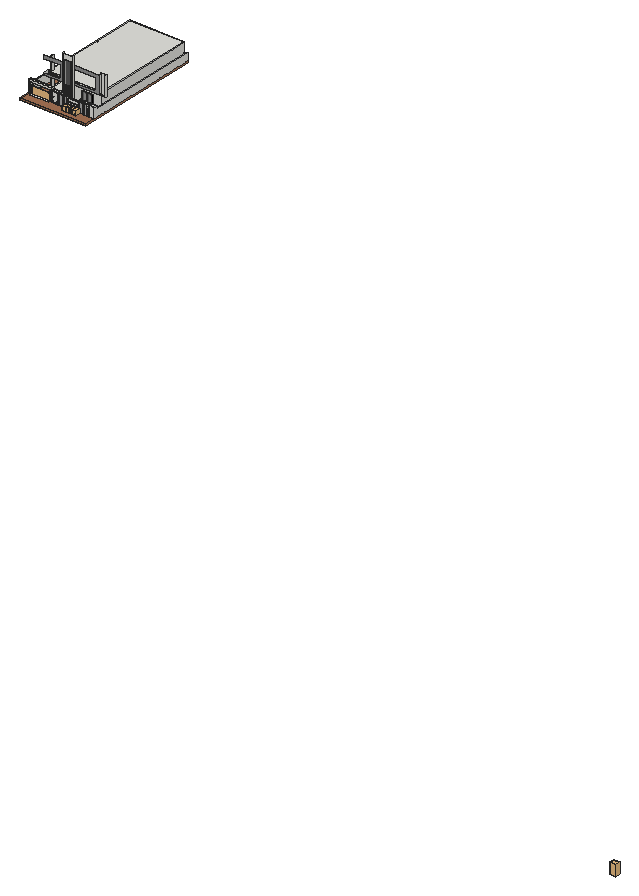
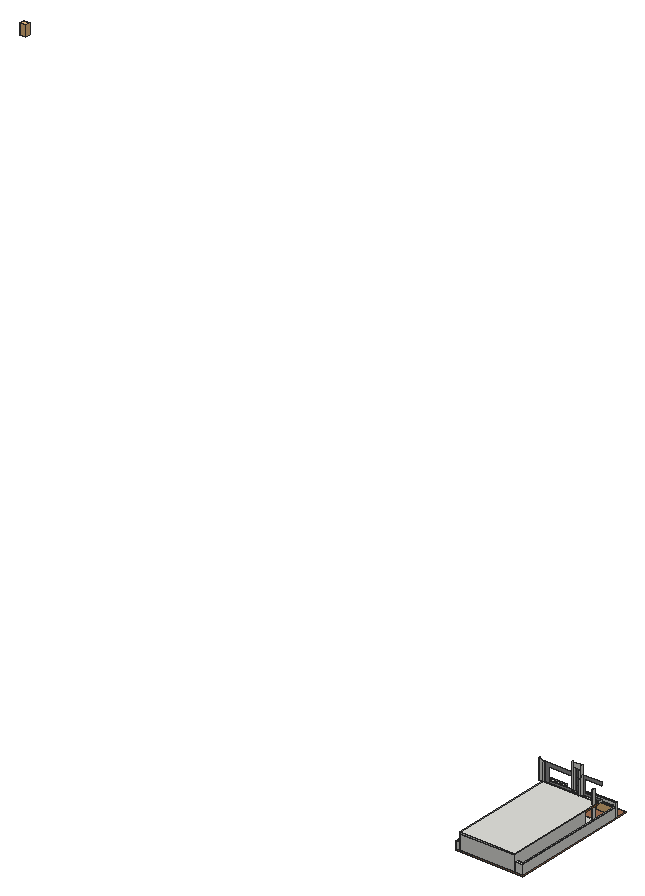
# SketchUp Ruby script. Lengths in inches.
U = 1.inch
M = Sketchup.active_model
def pt(a) = Geom::Point3d.new(a.map { |v| v * U })
def face(e, loops, mat)
  f = e.add_face(loops[0].map { |a| pt(a) })
  loops[1..].each { |l| e.add_face(l.map { |a| pt(a) }).erase! }
  f.material = f.back_material = mat if mat
  f
end
# faces: each face lists its corners as indices into pts; further lists are holes
def faces(e, pts, list, mat = nil) = list.each { |f| face(e, (f[0].is_a?(Array) ? f : [f]).map { |l| l.map { |i| pts[i] } }, mat) }
# xy, xz, yz: faces in a plane at the given z, y or x. An outline is a flat list of corners, or four numbers for a rectangle; further outlines are holes
def ring(l) = l.size == 4 ? [[l[0], l[1]], [l[2], l[1]], [l[2], l[3]], [l[0], l[3]]] : l.each_slice(2).to_a
def flat(e, list, mat, &to3) = list.each { |f| face(e, (f[0].is_a?(Array) ? f : [f]).map { |l| ring(l).map { |u, v| to3.(u, v) } }, mat) }
def xy(e, z, list, mat = nil) = flat(e, list, mat) { |x, y| [x, y, z] }
def xz(e, y, list, mat = nil) = flat(e, list, mat) { |x, z| [x, y, z] }
def yz(e, x, list, mat = nil) = flat(e, list, mat) { |y, z| [x, y, z] }
def lines(e, pts, list) = list.each { |a, b| e.add_line(pt(pts[a]), pt(pts[b])) }
# prism: a flat outline (further loops are holes) pulled along v
def prism(e, loops, v, mat = nil)
  f = face(e, loops, mat); d = Geom::Vector3d.new(v.map { |x| x * U })
  f.pushpull(f.normal.samedirection?(d) ? d.length : -d.length)
end
def box(e, o, s, mat = nil) = prism(e, [[o, [o[0] + s[0], o[1], o[2]], [o[0] + s[0], o[1] + s[1], o[2]], [o[0], o[1] + s[1], o[2]]]], [0, 0, s[2]], mat)
def at(x, y, z, deg = 0) = Geom::Transformation.translation(pt([x, y, z])) * Geom::Transformation.rotation(ORIGIN, Z_AXIS, deg.degrees)
def axes(o, x, y, z) = Geom::Transformation.new([*x, 0, *y, 0, *z, 0, *pt(o).to_a, 1])
def part(name) = M.definitions.add(name)
# library, detail: a bought-in or finely detailed component or shape, given as its bounding box
def library(name, o, s) = part(name).tap { |d| box(d.entities, o, s) }
def detail(e, o, s) = box(e.add_group.entities, o, s)
def put(e, d, t, mat = nil) = e.add_instance(d, t).tap { |i| i.material = mat if mat }
def group(e, t, mat = nil) = e.add_group.tap { |g| g.transformation = t; g.material = mat if mat }.entities
root = M.entities
M.materials.add("[Color B02]").color = [255, 178, 153]
M.materials.add("[Color M03]").color = [170, 170, 170]
M.materials.add("[Color M04]").color = [142, 142, 142]
M.materials.add("[Color M08]").color = [30, 30, 30]
M.materials.add("[Color_008]").color = [30, 30, 30]
M.materials.add("[Color_009]").color = [0, 0, 0]
M.materials.add("[Granite Dark Gray]").color = [69, 68, 68]
M.materials.add("[Tile Ceramic Multi]").color = [165, 115, 84]
M.materials.add("[Translucent Glass Gray]1").color = [128, 128, 128]
M.materials["[Translucent Glass Gray]1"].alpha = 0.5
M.materials.add("[Translucent_Glass_Gray]").color = [128, 128, 128]
M.materials["[Translucent_Glass_Gray]"].alpha = 0.5
M.materials.add("[Wood Bamboo]").color = [177, 105, 43]
c1 = library("climbing plant",[8874.76,-5589.78,-33.625],[50.13,38.07,87.16])
c2 = library("Slatted driveway gate",[-314.09,973.28,-346.04],[148.54,5.33,60.07])
c3 = part("Group\#12")
xz(c3.entities,0,[[0,0,51.1875,2.08]])
c4 = library("Broadleaf plant",[0,0,0],[149.19,166.1,98.1875])
c5 = part("Group\#13")
xz(c5.entities,0,[[0,0,45.4375,2.7]])
c6 = part("Janela")
xy(c6.entities,0,[[96.33,43.17,179.01,44.35]],"[Color_009]")
xy(c6.entities,1.97,[[98.3,44.15,136.6875,44.35],[138.66,44.15,177.04,44.35]])
xy(c6.entities,1.97,[[98.3,43.17,136.6875,43.46],[138.66,43.17,177.04,43.46]],"[Color_009]")
xy(c6.entities,80.71,[[98.3,43.17,136.6875,43.46],[138.66,43.17,177.04,43.46],[98.3,43.46,136.6875,44.15],[138.66,43.46,177.04,44.15],[98.3,44.15,136.6875,44.35],
  [138.66,44.15,177.04,44.35]])
xy(c6.entities,82.68,[[96.33,43.17,179.01,44.35]],"[Color_008]")
xz(c6.entities,43.17,[[[96.33,0,179.01,82.68],[98.3,1.97,136.6875,80.71],[138.66,1.97,177.04,80.71]]],"[Color_009]")
xz(c6.entities,43.46,[[98.3,1.97,136.6875,80.71],[138.66,1.97,177.04,80.71]],"[Translucent_Glass_Gray]")
xz(c6.entities,44.15,[[98.3,1.97,136.6875,80.71],[138.66,1.97,177.04,80.71]],"[Translucent_Glass_Gray]")
xz(c6.entities,44.35,[[[96.33,0,179.01,82.68],[98.3,1.97,177.04,80.71]],[136.6875,1.97,138.66,80.71]],"[Color_009]")
yz(c6.entities,96.33,[[43.17,0,44.35,82.68]],"[Color_009]")
yz(c6.entities,98.3,[[44.15,1.97,44.35,80.71]])
yz(c6.entities,98.3,[[43.17,1.97,43.46,80.71]],"[Color_009]")
yz(c6.entities,136.6875,[[43.17,1.97,43.46,80.71],[44.15,1.97,44.35,80.71]],"[Color_009]")
yz(c6.entities,138.66,[[43.17,1.97,43.46,80.71],[44.15,1.97,44.35,80.71]])
yz(c6.entities,177.04,[[43.17,1.97,43.46,80.71],[44.15,1.97,44.35,80.71]],"[Color_009]")
yz(c6.entities,179.01,[[43.17,0,44.35,82.68]],"[Color_009]")
c7 = library("Aluprof_MB-86_Drzwi_panelowe_003_S-0452",[0,0,0],[44.84,5.36,87])
c8 = part("Group\#15")
xz(c8.entities,0,[[0,0,96.8125,17.4]])
c9 = part("Group\#5")
box(c9.entities,[0,-1.25,0],[78.66,1.25,2.55])
c10 = part("Group\#6")
box(c10.entities,[0,-1.25,0],[15.54,1.25,1.96])
c11 = part("Group\#7")
box(c11.entities,[0,-1.25,0],[16.29,1.25,1.96])
c12 = part("Group\#10")
prism(c12.entities,[[[0,0.01,-2.4375],[0,129.01,-2.125],[7.8,129.01,-2.125],[7.8,0.01,-2.4375]]],[0,-0.01,2.4375])
xy(root,-0.4375,[[[316.25,46.4375,413.0625,87.8125],[320.83,51.02,408.48,83.23]],[320.83,51.02,408.48,83.23],[17.8125,71.9,174.3125,87.8125],[192.625,83.75,243.8125,107],[252.5625,83.75,280.625,107],
  [289.375,83.75,316.25,107],[413.0625,83.75,443.75,107],[452.5625,83.75,482.4375,107],[493.1875,83.75,493.1875,107,527.125,107,527.125,1033.27,506,1033.27,506,1045,538.625,1045,538.625,83.75],[0,87.8125,17.8125,104.375],
  [174.08,87.8125,192.625,104.375],[243.8125,87.8125,252.5625,107],[280.625,87.8125,289.375,107],[316.25,87.8125,413.0625,107],[443.75,87.8125,452.5625,107],
  [482.4375,87.8125,493.1875,107],[0,104.375,0,1045,62,1045,62,1019.26,13.64,1019.26,13.64,104.375],[[62,205,62,1045,505.75,1045,505.75,1033.27,506,1033.27,506,205],[71,214,497,214,497,518,353,518,353,338,349,338,349,522,397,522,397,582,349,582,349,758,418,758,418,806,373,806,373,936,237,936,237,864,183,864,183,734,179,734,179,800,71,800,71,526,239,526,239,730,243,730,243,522,219,522,219,338,71,338],[71,868,233,1036],[71,342,215,522],[353,586,497,754],[377,892,497,1036],[377,810,497,888],[301,940,373,1036],[71,804,179,864],[237,940,297,1036],[401,522,497,582],[422,758,497,806]],[505.75,1033.27,506,1045]])
xy(root,0,[[62,205,71,205,71,225.73,68.72,225.73,68.72,242.29,71,242.29,71,334,62,334],[71,205,215,205,215,214,497,214,497,334,71,334,71,242.29,82.03,242.29,82.03,225.73,71,225.73],[68.72,225.73,71,242.29],[71,225.73,82.03,242.29],[71,338,215,522],
  [219,338,349,338,349,522,397,522,397,582,349,582,349,758,418,758,418,806,373,806,373,936,237,936,237,864,183,864,183,734,243,734,243,522,219,522],[353,338,497,518],[401,522,497,582],[71,526,239,730],[353,586,497,754],
  [71,734,179,800],[422,758,497,806],[71,804,179,864],[377,810,497,888],[71,868,233,1036],
  [377,892,497,1036],[237,940,297,1036],[301,940,373,1036]])
xy(root,14.9375,[[[316.25,46.4375,413.0625,87.8125],[320.83,51.02,408.48,83.23]]],"[Granite Dark Gray]")
xy(root,15.25,[[215.24,166.5625,278.36,180.5],[278.36,166.5625,293.91,180.5]])
xy(root,59.14,[[527.125,107,538.625,107,538.625,1045,505.75,1045,505.75,1033.27,527.125,1033.27]])
xy(root,70.09,[[243.8125,87.8125,252.5625,107],[280.625,87.8125,289.375,107],[316.25,87.8125,413.0625,107],[443.75,87.8125,452.5625,107],[482.4375,87.8125,493.1875,107]])
xy(root,70.8125,[[0,104.375,13.64,104.375,13.64,1019.26,62,1019.26,62,1045,0,1045]])
xy(root,84.5,[[17.8125,87.8125,174.08,104.375]])
xy(root,86.1875,[[192.625,82.4375,243.8125,107],[252.5625,82.4375,280.625,83.75],[289.375,82.4375,316.25,83.75],[413.0625,82.4375,443.75,83.75],[452.5625,82.4375,482.4375,83.75],
  [493.1875,82.4375,493.1875,107,538.625,107,538.625,83.75,539.9375,83.75,539.9375,82.4375],[252.5625,83.75,280.625,107],[289.375,83.75,316.25,107],[413.0625,83.75,443.75,107],[452.5625,83.75,482.4375,107],
  [538.625,83.75,539.9375,107]])
xy(root,88.625,[[192.625,82.4375,243.8125,107],[413.0625,82.4375,443.75,107],[452.5625,82.4375,482.4375,107],[493.1875,82.4375,539.9375,107]])
xy(root,88.625,[[252.5625,82.4375,280.625,107],[289.375,82.4375,316.25,107]],"[Color M03]")
xy(root,104.5,[[0,87.8125,192.625,104.375]])
xy(root,105.54,[[231.53,166.5625,278.36,166.5625,278.36,180.5,254.95,180.5,254.95,176.36,252.06,176.36,252.06,180.5,231.53,180.5]])
xy(root,119.625,[[506,180.5,550.5625,195.0625]])
xy(root,119.6875,[[62,164.8125,215,205]])
xy(root,120,[[218,180.5,506,205],[[215,205,506,205,506,1045,62,1045,62,334,497,334,497,214,215,214],[219,338,219,522,243,522,243,730,239,730,239,526,71,526,71,800,179,800,179,734,183,734,183,864,237,864,237,936,373,936,373,806,418,806,418,758,349,758,349,582,397,582,397,522,349,522,349,338],[71,868,233,1036],[71,338,215,522],[353,338,497,518],[353,586,497,754],[377,892,497,1036],[377,810,497,888],[301,940,373,1036],[71,804,179,864],[237,940,297,1036],[401,522,497,582],[422,758,497,806]],[71,730,183,734],[183,730,243,734]])
xz(root,46.4375,[[316.25,-0.4375,413.0625,14.9375]],"[Granite Dark Gray]")
xz(root,51.02,[[320.83,-0.4375,408.48,14.9375]])
xz(root,82.4375,[[192.625,86.1875,243.8125,88.625],[493.1875,86.1875,539.9375,88.625]])
xz(root,82.4375,[[252.5625,86.1875,280.625,88.625],[289.375,86.1875,316.25,88.625],[413.0625,86.1875,443.75,88.625],[452.5625,86.1875,482.4375,88.625]],"[Color M03]")
xz(root,83.23,[[320.83,-0.4375,408.48,14.9375]],"[Granite Dark Gray]")
xz(root,83.75,[[192.625,-0.4375,243.8125,84.11],[493.1875,-0.4375,538.625,83.48]])
xz(root,83.75,[[252.5625,-0.4375,280.625,86.1875],[289.375,-0.4375,316.25,86.1875],[413.0625,-0.4375,443.75,86.1875],[452.5625,-0.4375,482.4375,86.1875]],"[Color M03]")
xz(root,87.8125,[[0,-0.4375,17.8125,-0.4375,17.8125,84.5,174.08,84.5,174.08,4.18,174.3125,4.18,174.3125,-0.4375,192.625,-0.4375,192.625,104.5,0,104.5],[17.8125,-0.4375,174.08,4.18],[174.08,-0.4375,174.3125,4.18],[243.8125,-0.4375,252.5625,70.09],[280.625,-0.4375,289.375,70.09],
  [316.25,-0.4375,413.0625,14.9375],[443.75,-0.4375,452.5625,70.09],[482.4375,-0.4375,493.1875,70.09],[316.25,14.9375,413.0625,52.69]])
xz(root,104.375,[[13.64,-0.4375,13.64,70.8125,0,70.8125,0,104.5,192.625,104.5,192.625,-0.4375,174.08,-0.4375,174.08,84.5,17.8125,84.5,17.8125,-0.4375]])
xz(root,107,[[192.625,-0.4375,243.8125,86.1875],[243.8125,-0.4375,252.5625,70.09],[252.5625,-0.4375,280.625,86.1875],[280.625,-0.4375,289.375,70.09],[289.375,-0.4375,316.25,86.1875],
  [316.25,-0.4375,413.0625,70.09],[413.0625,-0.4375,443.75,86.1875],[443.75,-0.4375,452.5625,70.09],[452.5625,-0.4375,482.4375,86.1875],[482.4375,-0.4375,493.1875,70.09],
  [493.1875,-0.4375,527.125,86.1875],[527.125,59.14,538.625,86.1875],[192.625,86.1875,243.8125,88.625],[252.5625,86.1875,280.625,88.625],[289.375,86.1875,316.25,88.625],
  [413.0625,86.1875,443.75,88.625],[452.5625,86.1875,482.4375,88.625],[493.1875,86.1875,539.9375,88.625]])
xz(root,164.8125,[[62,119.6875,215,119.6875,215,264.4375,62,264.4375,62,237,199.16,237,199.16,135.79,62,135.79]],"[Color M04]")
xz(root,165.3125,[[231.53,107.81,278.36,291.73]],"[Translucent Glass Gray]1")
xz(root,166.5625,[[215.24,15.25,278.36,15.25,278.36,105.54,231.53,105.54,231.53,289.77,215.24,289.77],[278.36,15.25,293.91,15.25,293.91,332.01,215.24,332.01,215.24,291.73,231.53,291.73,231.53,292.78,278.36,292.78]])
xz(root,176.36,[[252.06,105.54,254.95,292.39]],"[Color M08]")
xz(root,180.5,[[218,15.25,218,120,231.53,120,231.53,105.54,252.06,105.54,252.06,120,254.95,120,254.95,105.54,278.36,105.54,278.36,15.25],[278.36,15.25,293.91,120],[506,119.625,550.5625,132.38],[218,120,231.53,136.625],[231.53,120,252.06,136.625],
  [252.06,120,254.95,136.625],[254.95,120,278.36,136.625],[278.36,120,293.91,136.625]])
xz(root,180.5,[[293.91,120,506,120,506,264.4375,293.91,264.4375,293.91,237,473.75,237,473.75,136.625,293.91,136.625]],"[Color M04]")
xz(root,180.5,[[215.24,15.25,215.24,237,252.06,237,252.06,233.875,231.53,233.875,231.53,180.8125,252.06,180.8125,252.06,175.4375,231.53,175.4375,231.53,136.625,218,136.625,218,15.25]],"[Color M08]")
xz(root,195.0625,[[506,119.625,550.5625,277.75]])
xz(root,205,[[62,-0.4375,506,-0.4375,506,120,215,120,215,0,62,0],[62,119.6875,215,132],[218,120,506,132]])
xz(root,214,[[215,0,497,120]])
xz(root,225.73,[[68.72,0,82.03,235.5625]])
xz(root,242.29,[[68.72,0,82.03,235.5625]])
xz(root,334,[[62,0,71,120]])
xz(root,334,[[71,0,497,120]],"[Color B02]")
xz(root,338,[[71,0,215,120],[219,0,349,120],[353,0,497,120]])
xz(root,518,[[353,-0.4375,497,0],[353,0,497,120]])
xz(root,522,[[71,-0.4375,215,0],[219,-0.4375,243,0],[349,-0.4375,397,0],[401,-0.4375,497,0],[71,0,215,120],
  [219,0,243,120],[349,0,397,120],[401,0,497,120]])
xz(root,526,[[71,-0.4375,239,0],[71,0,239,120]])
xz(root,582,[[349,-0.4375,397,0],[401,-0.4375,497,0],[349,0,397,120],[401,0,497,120]])
xz(root,586,[[353,-0.4375,497,0],[353,0,497,120]])
xz(root,730,[[239,-0.4375,243,120],[71,0,183,120],[183,0,239,120]])
xz(root,734,[[179,-0.4375,183,120],[71,0,179,120],[183,0,243,120]])
xz(root,754,[[353,-0.4375,497,0],[353,0,497,120]])
xz(root,758,[[349,-0.4375,418,0],[422,-0.4375,497,0],[349,0,418,120],[422,0,497,120]])
xz(root,800,[[71,-0.4375,179,0],[71,0,179,120]])
xz(root,804,[[71,-0.4375,179,0],[71,0,179,120]])
xz(root,806,[[373,-0.4375,418,0],[422,-0.4375,497,0],[373,0,418,120],[422,0,497,120]])
xz(root,810,[[377,-0.4375,497,0],[377,0,497,120]])
xz(root,864,[[71,-0.4375,179,0],[183,-0.4375,237,0],[71,0,179,120],[183,0,237,120]])
xz(root,868,[[71,-0.4375,233,0],[71,0,233,120]])
xz(root,888,[[377,-0.4375,497,0],[377,0,497,120]])
xz(root,892,[[377,-0.4375,497,0],[377,0,497,120]])
xz(root,936,[[237,-0.4375,373,0],[237,0,373,120]])
xz(root,940,[[237,-0.4375,297,0],[301,-0.4375,373,0],[237,0,297,120],[301,0,373,120]])
xz(root,1019.26,[[13.64,-0.4375,62,70.8125]])
xz(root,1033.27,[[505.75,-0.4375,527.125,59.14]])
xz(root,1036,[[71,-0.4375,233,0],[237,-0.4375,297,0],[301,-0.4375,373,0],[377,-0.4375,497,0],[71,0,233,120],
  [237,0,297,120],[301,0,373,120],[377,0,497,120]])
xz(root,1045,[[0,-0.4375,62,70.8125],[62,-0.4375,62,120,506,120,506,59.14,505.75,59.14,505.75,-0.4375],[505.75,-0.4375,506,59.14],[506,-0.4375,538.625,59.14]])
yz(root,0,[[87.8125,-0.4375,104.375,104.5],[104.375,-0.4375,1045,70.8125]])
yz(root,13.64,[[104.375,-0.4375,1019.26,70.8125]])
yz(root,17.8125,[[71.9,-0.4375,87.8125,4.18,87.8125,-0.4375],[87.8125,-0.4375,104.375,84.5]])
yz(root,62,[[205,-0.4375,205,0,334,0,334,120,1045,120,1045,70.8125,1019.26,70.8125,1019.26,-0.4375],[1019.26,-0.4375,1045,70.8125],[164.8125,119.6875,205,135.79]])
yz(root,68.72,[[225.73,0,242.29,235.5625]])
yz(root,71,[[342,-0.4375,522,0],[526,-0.4375,730,0],[730,-0.4375,734,120],[734,-0.4375,800,0],[804,-0.4375,864,0],
  [868,-0.4375,1036,0],[338,0,342,120],[342,0,522,120],[526,0,730,120],[734,0,800,120],
  [804,0,864,120],[868,0,1036,120]])
yz(root,82.03,[[225.73,0,242.29,235.5625]])
yz(root,174.08,[[87.8125,-0.4375,104.375,84.5]])
yz(root,174.3125,[[71.9,-0.4375,87.8125,-0.4375,87.8125,4.18]])
yz(root,179,[[734,-0.4375,800,0],[804,-0.4375,864,0],[734,0,800,120],[804,0,864,120]])
yz(root,183,[[734,-0.4375,864,0],[734,0,864,120]])
yz(root,192.625,[[83.75,-0.4375,87.8125,86.1875],[87.8125,-0.4375,104.375,86.1875],[104.375,-0.4375,107,86.1875],[82.4375,86.1875,87.8125,88.625],[87.8125,86.1875,104.375,88.625],
  [104.375,86.1875,107,88.625],[87.8125,88.625,104.375,104.5]])
yz(root,215,[[342,-0.4375,522,0],[205,0,214,120],[338,0,342,120],[342,0,522,120],[164.8125,119.6875,180.5,264.4375],
  [180.5,119.6875,205,237]])
yz(root,215.24,[[166.5625,15.25,180.5,334.5625]])
yz(root,218,[[180.5,120,205,136.625]])
yz(root,219,[[338,-0.4375,522,0],[338,0,522,120]])
yz(root,231.53,[[166.5625,105.54,180.5,105.54,180.5,175.4375,173.5625,175.4375,173.5625,180.8125,180.5,180.8125,180.5,233.875,172.8125,233.875,172.8125,237,180.5,237,180.5,292.78,166.5625,292.78]])
yz(root,233,[[868,-0.4375,1036,0],[868,0,1036,120]])
yz(root,237,[[864,-0.4375,936,0],[940,-0.4375,1036,0],[864,0,936,120],[940,0,1036,120]])
yz(root,239,[[526,-0.4375,730,0],[526,0,730,120]])
yz(root,243,[[522,-0.4375,730,0],[522,0,730,120],[730,0,734,120]])
yz(root,243.8125,[[83.75,-0.4375,87.8125,70.09],[87.8125,-0.4375,107,70.09],[83.75,70.09,107,86.1875],[82.4375,86.1875,107,88.625]])
yz(root,252.06,[[176.36,105.54,180.5,292.39]])
yz(root,252.5625,[[83.75,-0.4375,87.8125,70.09],[87.8125,-0.4375,107,70.09],[83.75,70.09,107,86.1875],[82.4375,86.1875,107,88.625]])
yz(root,254.95,[[176.36,105.54,180.5,292.39]],"[Color M08]")
yz(root,278.36,[[166.5625,15.25,180.5,105.54],[166.5625,105.54,166.5625,292.78,180.5,292.78,180.5,180.8125,173.5625,180.8125,173.5625,175.4375,180.5,175.4375,180.5,105.54]])
yz(root,280.625,[[83.75,-0.4375,87.8125,70.09],[87.8125,-0.4375,107,70.09],[83.75,70.09,107,86.1875],[82.4375,86.1875,107,88.625]])
yz(root,289.375,[[83.75,-0.4375,87.8125,70.09],[87.8125,-0.4375,107,70.09],[83.75,70.09,107,86.1875],[82.4375,86.1875,107,88.625]])
yz(root,293.91,[[166.5625,15.25,180.5,334.5625]])
yz(root,297,[[940,-0.4375,1036,0],[940,0,1036,120]])
yz(root,301,[[940,-0.4375,1036,0],[940,0,1036,120]])
yz(root,316.25,[[83.75,-0.4375,87.8125,14.9375],[87.8125,-0.4375,107,70.09],[83.75,14.9375,87.8125,70.09],[83.75,70.09,107,86.1875],[82.4375,86.1875,107,88.625]])
yz(root,316.25,[[46.4375,-0.4375,83.75,14.9375]],"[Granite Dark Gray]")
yz(root,320.83,[[51.02,-0.4375,83.23,14.9375]],"[Granite Dark Gray]")
yz(root,349,[[338,-0.4375,522,0],[582,-0.4375,758,0],[338,0,522,120],[582,0,758,120]])
yz(root,353,[[338,-0.4375,518,0],[586,-0.4375,754,0],[338,0,518,120],[586,0,754,120]])
yz(root,373,[[806,-0.4375,936,0],[940,-0.4375,1036,0],[806,0,936,120],[940,0,1036,120]])
yz(root,377,[[810,-0.4375,888,0],[892,-0.4375,1036,0],[810,0,888,120],[892,0,1036,120]])
yz(root,397,[[522,-0.4375,582,0],[522,0,582,120]])
yz(root,401,[[522,-0.4375,582,0],[522,0,582,120]])
yz(root,408.48,[[51.02,-0.4375,83.23,14.9375]],"[Granite Dark Gray]")
yz(root,413.0625,[[83.75,-0.4375,87.8125,14.9375],[87.8125,-0.4375,107,70.09],[83.75,14.9375,87.8125,70.09],[83.75,70.09,107,86.1875],[82.4375,86.1875,107,88.625]])
yz(root,413.0625,[[46.4375,-0.4375,83.75,14.9375]],"[Granite Dark Gray]")
yz(root,418,[[758,-0.4375,806,0],[758,0,806,120]])
yz(root,422,[[758,-0.4375,806,0],[758,0,806,120]])
yz(root,443.75,[[83.75,-0.4375,87.8125,70.09],[87.8125,-0.4375,107,70.09],[83.75,70.09,107,86.1875],[82.4375,86.1875,107,88.625]])
yz(root,452.5625,[[83.75,-0.4375,87.8125,70.09],[87.8125,-0.4375,107,70.09],[83.75,70.09,107,86.1875]])
yz(root,452.5625,[[82.4375,86.1875,107,88.625]],"[Color M03]")
yz(root,482.4375,[[83.75,-0.4375,87.8125,70.09],[87.8125,-0.4375,107,70.09],[83.75,70.09,107,86.1875],[82.4375,86.1875,107,88.625]])
yz(root,493.1875,[[83.75,-0.4375,87.8125,70.09],[87.8125,-0.4375,107,70.09],[83.75,70.09,107,86.1875],[82.4375,86.1875,107,88.625]])
yz(root,497,[[338,-0.4375,518,0],[522,-0.4375,582,0],[586,-0.4375,754,0],[758,-0.4375,806,0],[810,-0.4375,888,0],
  [892,-0.4375,1036,0],[214,0,334,120],[338,0,518,120],[522,0,582,120],[586,0,754,120],
  [758,0,806,120],[810,0,888,120],[892,0,1036,120]])
yz(root,505.75,[[1033.27,-0.4375,1045,59.14]])
yz(root,506,[[205,-0.4375,1045,120],[180.5,119.625,195.0625,120],[180.5,120,195.0625,120,195.0625,264.4375,182.5,264.4375,182.5,264.38,180.5,264.38,180.5,255.38,182.5,255.38,182.5,253.38,180.5,253.38,180.5,244.38,182.5,244.38,182.5,242.38,180.5,242.38,180.5,233.38,182.5,233.38,182.5,231.38,180.5,231.38,180.5,222.38,182.5,222.38,182.5,220.38,180.5,220.38,180.5,211.38,182.5,211.38,182.5,209.38,180.5,209.38,180.5,200.38,182.5,200.38,182.5,198.38,180.5,198.38,180.5,189.38,182.5,189.38,182.5,187.38,180.5,187.38,180.5,178.38,182.5,178.38,182.5,176.38,180.5625,176.38,180.5625,167.38,182.5625,167.38,182.5625,165.38,180.5,165.38,180.5,156.38,182.5,156.38,182.5,154.38,180.5,154.38,180.5,145.38,182.5,145.38,182.5,143.38,180.5,143.38,180.5,134.38,182.5,134.38,182.5,132.38,180.5,132.38],[195.0625,120,205,264.4375]])
yz(root,527.125,[[107,-0.4375,1033.27,59.14]])
yz(root,538.625,[[83.75,-0.4375,1045,-0.4375,1045,59.14,107,59.14,107,86.1875,83.75,86.1875]])
yz(root,539.9375,[[82.4375,86.1875,107,88.625]])
yz(root,550.5625,[[180.5,119.625,195.0625,119.625,195.0625,277.75,180.5,277.75,180.5,266.38,182.5,266.38,182.5,264.38,180.5,264.38,180.5,255.38,182.5,255.38,182.5,253.38,180.5,253.38,180.5,244.38,182.5,244.38,182.5,242.38,180.5,242.38,180.5,233.38,182.5,233.38,182.5,231.38,180.5,231.38,180.5,222.38,182.5,222.38,182.5,220.38,180.5,220.38,180.5,211.38,182.5,211.38,182.5,209.38,180.5,209.38,180.5,200.38,182.5,200.38,182.5,198.38,180.5,198.38,180.5,189.38,182.5,189.38,182.5,187.38,180.5,187.38,180.5,178.38,182.5,178.38,182.5,176.38,180.5625,176.38,180.5625,167.38,182.5625,167.38,182.5625,165.38,180.5,165.38,180.5,156.38,182.5,156.38,182.5,154.38,180.5,154.38,180.5,145.38,182.5,145.38,182.5,143.38,180.5,143.38,180.5,134.38,182.5,134.38,182.5,132.38,180.5,132.38]])
p = [[17.8125,87.8125,4.18],[17.8125,71.9,-0.4375],[174.3125,71.9,-0.4375],[174.3125,87.8125,4.18],[174.08,87.8125,4.18],[497,214,0],
  [497,214,-0.4375],[71,214,0],[71,214,-0.4375],[71,338,0],[71,338,-0.4375]]
faces(root,p,[[0,1,2,3,4]])
lines(root,p,[[5,6],[7,8],[9,10]])
put(root,c1,at(352.56,83.23,6.31))
g1 = group(root,at(62,1045,-12.4375),"[Tile Ceramic Multi]")
box(g1,[-62,-1045,0],[538.625,1045,12])
g2 = group(root,at(316.25,87.8125,-5.64))
xz(g2,0,[[0,0,96.8125,17.4]])
put(root,c2,at(336.08,-885.47,345.6))
put(root,c3,at(192.625,83.75,-0.4375))
put(root,c4,axes([308.41,43.03,-0.4375],[0.3456,0,0],[0,0.3456,0],[0,0,0.3456]))
put(root,c4,axes([338.22,43.03,-0.4375],[0.3456,0,0],[0,0.3456,0],[0,0,0.3456]))
put(root,c4,axes([369.03,43.03,-0.4375],[0.3456,0,0],[0,0.3456,0],[0,0,0.3456]))
put(root,c5,at(493.1875,83.75,2.55))
put(root,c3,at(192.625,83.75,3.78))
put(root,c6,at(250.89,157.54,4.82))
put(root,c7,axes([192.06,328.64,5.64],[1,0,0],[0,1,0],[0,0,0.89]))
put(root,c3,at(192.625,83.75,7.16))
put(root,c5,at(493.1875,83.75,7.36))
put(root,c3,at(192.625,83.75,10.91))
put(root,c5,at(493.1875,83.75,11.98))
put(root,c3,at(192.625,83.75,14.09))
put(root,c8,at(316.25,87.8125,14.67))
put(root,c5,at(493.1875,83.75,16.11))
put(root,c9,at(215.24,166.5625,16.46))
put(root,c3,at(192.625,83.75,17.84))
put(root,c9,at(215.24,166.5625,19.39))
put(root,c5,at(493.1875,83.75,20.55))
put(root,c3,at(192.625,83.75,21.53))
put(root,c9,at(215.24,166.5625,22.21))
put(root,c5,at(493.1875,83.75,25.05))
put(root,c3,at(192.625,83.75,25.22))
put(root,c9,at(215.24,166.5625,25.33))
put(root,c9,at(215.24,166.5625,28.52))
put(root,c3,at(192.625,83.75,28.59))
put(root,c5,at(493.1875,83.75,29.42))
put(root,c9,at(215.24,166.5625,31.58))
put(root,c3,at(192.625,83.75,32.28))
put(root,c8,at(316.25,87.8125,33.73))
put(root,c5,at(493.1875,83.75,34.05))
put(root,c9,at(215.24,166.5625,34.64))
put(root,c3,at(192.625,83.75,36.16))
put(root,c9,at(215.24,166.5625,37.71))
put(root,c5,at(493.1875,83.75,38.61))
put(root,c3,at(192.625,83.75,39.66))
put(root,c9,at(215.24,166.5625,40.64))
put(root,c5,at(493.1875,83.75,43.11))
put(root,c3,at(192.625,83.75,43.34))
put(root,c9,at(215.24,166.5625,43.89))
put(root,c9,at(215.24,166.5625,46.96))
put(root,c3,at(192.625,83.75,47.16))
put(root,c5,at(493.1875,83.75,47.3))
put(root,c9,at(215.24,166.5625,50.08))
put(root,c3,at(192.625,83.75,50.91))
put(root,c5,at(493.1875,83.75,51.73))
put(root,c8,at(316.25,87.8125,52.69))
put(root,c9,at(215.24,166.5625,53.02))
put(root,c3,at(192.625,83.75,54.78))
put(root,c5,at(493.1875,83.75,55.92))
put(root,c9,at(215.24,166.5625,55.96))
put(root,c3,at(192.625,83.75,58.66))
put(root,c9,at(215.24,166.5625,58.89))
put(root,c5,at(493.1875,83.75,59.73))
put(root,c9,at(215.24,166.5625,61.89))
put(root,c3,at(192.625,83.75,62.47))
put(root,c5,at(493.1875,83.75,63.36))
put(root,c9,at(215.24,166.5625,64.71))
put(root,c3,at(192.625,83.75,66.28))
put(root,c5,at(493.1875,83.75,67.17))
put(root,c9,at(215.24,166.5625,67.71))
put(root,c3,at(192.625,83.75,70.09))
put(root,c9,at(215.24,166.5625,70.64))
put(root,c5,at(493.1875,83.75,71.3))
put(root,c9,at(215.24,166.5625,73.52))
put(root,c3,at(192.625,83.75,73.72))
put(root,c5,at(493.1875,83.75,75.36))
put(root,c9,at(215.24,166.5625,76.52))
put(root,c3,at(192.625,83.75,77.1))
put(root,c5,at(493.1875,83.75,79.36))
put(root,c9,at(215.24,166.5625,79.52))
put(root,c3,at(192.625,83.75,80.42))
put(root,c9,at(215.24,166.5625,82.95))
put(root,c5,at(493.1875,83.75,83.48))
put(root,c3,at(192.625,83.75,84.11))
put(root,c9,at(215.24,166.5625,86.39))
put(root,c9,at(215.24,166.5625,89.64))
put(root,c9,at(215.24,166.5625,92.95))
put(root,c9,at(215.24,166.5625,96.01))
put(root,c9,at(215.24,166.5625,99.39))
put(root,c9,at(215.24,166.5625,102.95))
put(root,c10,at(278.36,166.5625,105.85))
put(root,c11,at(215.24,166.5625,106.09))
put(root,c10,at(278.36,166.5625,108.41))
put(root,c11,at(215.24,166.5625,108.77))
put(root,c10,at(278.36,166.5625,110.85))
put(root,c11,at(215.24,166.5625,111.27))
put(root,c10,at(278.36,166.5625,113.22))
put(root,c11,at(215.24,166.5625,113.71))
put(root,c10,at(278.36,166.5625,115.97))
put(root,c11,at(215.24,166.5625,116.27))
put(root,c12,at(62,205,119.6875),"[Wood Bamboo]")
put(root,c12,at(72.0625,205,119.6875),"[Wood Bamboo]")
put(root,c12,at(81.125,204.99,119.6875),"[Wood Bamboo]")
put(root,c12,at(90.75,204.99,119.6875),"[Wood Bamboo]")
put(root,c12,at(100.16,204.99,119.6875),"[Wood Bamboo]")
put(root,c12,at(109.53,204.99,119.6875),"[Wood Bamboo]")
put(root,c12,at(119.53,204.99,119.6875),"[Wood Bamboo]")
put(root,c12,at(129.35,204.99,119.6875),"[Wood Bamboo]")
put(root,c12,at(138.85,204.99,119.6875),"[Wood Bamboo]")
put(root,c12,at(148.6,204.99,119.6875),"[Wood Bamboo]")
put(root,c12,at(157.85,204.99,119.6875),"[Wood Bamboo]")
put(root,c12,at(167.53,204.99,119.6875),"[Wood Bamboo]")
put(root,c12,at(176.78,204.99,119.6875),"[Wood Bamboo]")
put(root,c12,at(186.53,204.99,119.6875),"[Wood Bamboo]")
put(root,c12,at(196.1,204.99,119.6875),"[Wood Bamboo]")
put(root,c12,at(205.16,204.99,119.6875),"[Wood Bamboo]")
put(root,c12,at(214.41,204.99,119.6875),"[Wood Bamboo]")
put(root,c12,at(223.91,204.99,119.6875),"[Wood Bamboo]")
put(root,c11,at(215.24,166.5625,118.71))
put(root,c10,at(278.36,166.5625,119.1))
g3 = group(root,at(62,1045,120))
box(g3,[0,-840,0],[444,840,12])
put(root,c11,at(215.24,166.5625,121.15))
put(root,c10,at(278.36,166.5625,121.78))
put(root,c11,at(215.24,166.5625,123.59))
put(root,c10,at(278.36,166.5625,124.47))
put(root,c11,at(215.24,166.5625,125.84))
put(root,c10,at(278.36,166.5625,127.03))
put(root,c11,at(215.24,166.5625,128.15))
put(root,c10,at(278.36,166.5625,129.6))
put(root,c11,at(215.24,166.5625,130.59))
